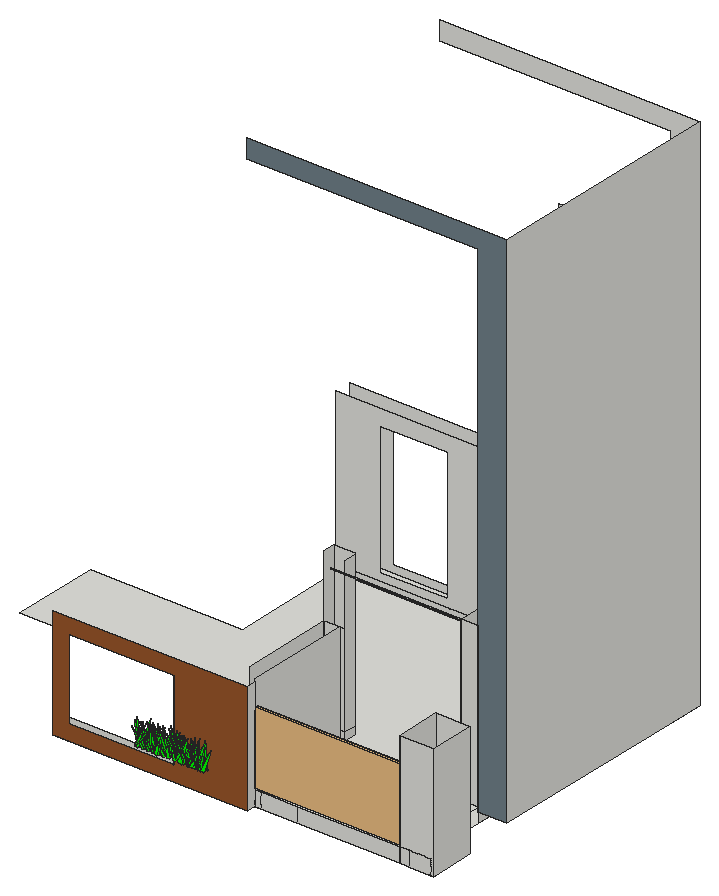
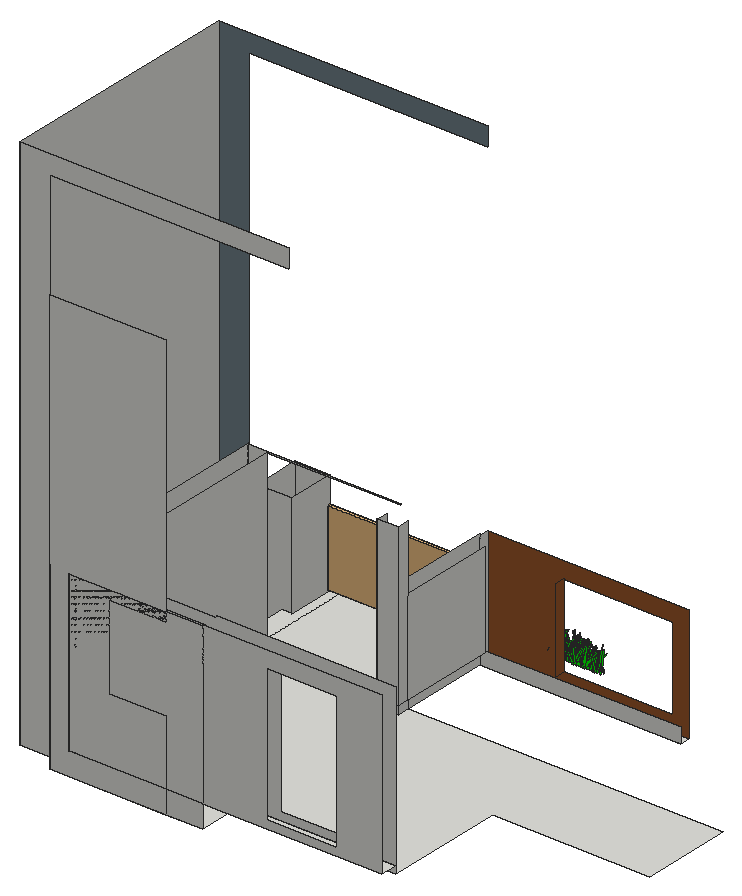
# SketchUp Ruby script. Lengths in inches.
U = 1.inch
M = Sketchup.active_model
def pt(a) = Geom::Point3d.new(a.map { |v| v * U })
def face(e, loops, mat)
  f = e.add_face(loops[0].map { |a| pt(a) })
  loops[1..].each { |l| e.add_face(l.map { |a| pt(a) }).erase! }
  f.material = f.back_material = mat if mat
  f
end
# faces: each face lists its corners as indices into pts; further lists are holes
def faces(e, pts, list, mat = nil) = list.each { |f| face(e, (f[0].is_a?(Array) ? f : [f]).map { |l| l.map { |i| pts[i] } }, mat) }
# xy, xz, yz: faces in a plane at the given z, y or x. An outline is a flat list of corners, or four numbers for a rectangle; further outlines are holes
def ring(l) = l.size == 4 ? [[l[0], l[1]], [l[2], l[1]], [l[2], l[3]], [l[0], l[3]]] : l.each_slice(2).to_a
def flat(e, list, mat, &to3) = list.each { |f| face(e, (f[0].is_a?(Array) ? f : [f]).map { |l| ring(l).map { |u, v| to3.(u, v) } }, mat) }
def xy(e, z, list, mat = nil) = flat(e, list, mat) { |x, y| [x, y, z] }
def xz(e, y, list, mat = nil) = flat(e, list, mat) { |x, z| [x, y, z] }
def yz(e, x, list, mat = nil) = flat(e, list, mat) { |y, z| [x, y, z] }
def lines(e, pts, list) = list.each { |a, b| e.add_line(pt(pts[a]), pt(pts[b])) }
# prism: a flat outline (further loops are holes) pulled along v
def prism(e, loops, v, mat = nil)
  f = face(e, loops, mat); d = Geom::Vector3d.new(v.map { |x| x * U })
  f.pushpull(f.normal.samedirection?(d) ? d.length : -d.length)
end
def box(e, o, s, mat = nil) = prism(e, [[o, [o[0] + s[0], o[1], o[2]], [o[0] + s[0], o[1] + s[1], o[2]], [o[0], o[1] + s[1], o[2]]]], [0, 0, s[2]], mat)
def at(x, y, z, deg = 0) = Geom::Transformation.translation(pt([x, y, z])) * Geom::Transformation.rotation(ORIGIN, Z_AXIS, deg.degrees)
def axes(o, x, y, z) = Geom::Transformation.new([*x, 0, *y, 0, *z, 0, *pt(o).to_a, 1])
def part(name) = M.definitions.add(name)
# library, detail: a bought-in or finely detailed component or shape, given as its bounding box
def library(name, o, s) = part(name).tap { |d| box(d.entities, o, s) }
def detail(e, o, s) = box(e.add_group.entities, o, s)
def put(e, d, t, mat = nil) = e.add_instance(d, t).tap { |i| i.material = mat if mat }
def group(e, t, mat = nil) = e.add_group.tap { |g| g.transformation = t; g.material = mat if mat }.entities
root = M.entities
M.materials.add("[0065_Lime]").color = [0, 255, 0]
M.materials.add("[0111_SlateGray]1").color = [112, 128, 136]
M.materials.add("[Wood Cherry Original]").color = [152, 86, 42]
c1 = part("fur_instance\#9")
p = [[0.8125,0,1.79],[0.67,-0.02,1.48],[0,-0.11,0],[0,0.11,0]]
faces(c1.entities,p,[[0,1,2,3]])
c2 = library("Modern+Gate+1",[0,0,0],[118.11,1.97,78.74])
xy(root,-11.8125,[[187.77,39.75,190.59,97.05],[190.59,39.75,210.17,217.05],[210.17,39.75,210.17,217.05,270.7,217.05,270.7,64.5,265.92,64.5,265.92,39.75],[265.92,39.75,270.7,64.5],[270.7,39.75,284.23,64.5]])
xy(root,-11.6,[[82.49,34.4375,187.77,39.75]])
xy(root,-6,[[270.7,86.99,286.33,217.05]])
xy(root,-3.9375,[[187.77,39.75,260.82,39.75,260.82,208.05,96.96,208.05,96.96,144.8,14.71,144.8,14.71,97.05,179.21,97.05,179.21,103.41,190.59,103.41,190.59,97.05,187.77,97.05],[260.82,39.75,270.7,87.55]])
xy(root,0,[[179.21,97.05,190.59,103.41],[96.96,208.05,190.59,217.05],[190.59,208.05,260.82,217.05]])
xz(root,34.4375,[[[82.49,-11.6,187.77,48.65],[90.86,-3.22,147.74,40.28]]],"[Wood Cherry Original]")
xz(root,39.75,[[187.77,-11.8125,190.59,-3.9375],[190.59,-11.8125,210.17,-3.9375],[210.17,-11.8125,265.92,-3.9375],[265.92,-11.8125,270.7,-3.9375],[282.96,-11.8125,284.23,-11.8125,284.23,49.9375,265.92,49.9375,265.92,-3.9375,282.96,-3.9375],
  [270.7,-11.8125,282.96,-3.9375],[82.49,-11.6,187.77,-3.9375]])
xz(root,64.5,[[265.92,-11.8125,284.23,49.9375]])
xz(root,86.99,[[270.7,-6,286.33,-6,286.33,276.75,145.58,276.75,145.58,266.9,270.7,266.9]],"[0111_SlateGray]1")
xz(root,87.55,[[260.82,-3.9375,270.7,-3.9375,270.7,84,190.59,84,190.59,83.3,260.82,83.3]])
xz(root,97.05,[[187.77,-11.8125,190.59,-3.9375],[187.77,-3.9375,190.59,0],[179.21,0,187.77,49.9375],[187.77,0,190.59,49.9375]])
xz(root,103.41,[[179.21,-3.9375,190.59,0],[179.21,0,190.59,84]])
xz(root,208.05,[[96.96,-3.9375,190.59,0],[190.59,-3.9375,260.82,0],[[96.96,0,260.82,0,260.82,83.3,190.59,83.3,190.59,84,96.96,84],[120.48,4.04,157.11,75.48],[195.64,34.28,239.77,78.41]]])
xz(root,217.05,[[190.59,-11.8125,210.17,0],[210.17,-11.8125,210.17,0,260.82,0,260.82,83.3,210.17,83.3,210.17,210.6875,270.7,210.6875,270.7,-11.8125],[270.7,-6,270.7,266.9,145.58,266.9,145.58,276.75,286.33,276.75,286.33,-6],[[96.96,0,190.59,84],[120.48,4.04,157.11,75.48]],[190.59,0,260.82,83.3],
  [210.17,0,210.17,34.28,239.77,34.28,239.77,78.41,210.17,78.41,210.17,83.3,260.82,83.3,260.82,0]])
yz(root,147.74,[[34.4375,-3.22,39.75,40.28]],"[Wood Cherry Original]")
yz(root,179.21,[[97.05,-3.9375,103.41,0],[46.62,0,97.05,49.9375],[97.05,0,103.41,84]])
yz(root,187.77,[[39.75,-11.8125,97.05,-3.9375],[34.4375,-11.6,39.75,48.65],[39.75,-3.9375,97.05,49.9375]])
yz(root,190.59,[[97.05,-3.9375,103.41,0],[97.05,0,103.41,83.3]])
yz(root,260.82,[[87.55,-3.9375,208.05,83.3],[208.05,0,217.05,83.3]])
yz(root,265.92,[[39.75,-11.8125,64.5,49.9375]])
yz(root,270.7,[[87.55,-11.8125,217.05,-6],[86.99,-6,217.05,-6,217.05,84,87.55,84,87.55,-3.9375,86.99,-3.9375],[86.99,-3.9375,87.55,84]])
yz(root,284.23,[[39.75,-11.8125,64.5,49.9375]])
yz(root,286.33,[[86.99,-6,217.05,276.75]])
put(root,c1,axes([131.16,30.08,1.48],[1.34479,0.85676,0.05361],[-5.98551,0.18367,0.98068],[1.16348,-0.04536,4.98315]),"[0065_Lime]")
put(root,c1,axes([154.34,30.49,1.48],[3.14543,1.05905,2.9173],[-8.27321,0.32433,1.95662],[1.10444,-0.58664,6.34829]),"[0065_Lime]")
put(root,c1,axes([151.13,30.3,1.48],[1.80183,0.66729,0.2231],[-4.17247,0.20193,2.05746],[2.28398,-0.15752,3.58266]),"[0065_Lime]")
put(root,c1,axes([145.91,30.29,1.48],[-2.59905,0.85083,0.56619],[-5.79357,-0.31187,-1.89204],[-1.89246,-0.21373,5.01467]),"[0065_Lime]")
put(root,c1,axes([159.01,30.73,1.48],[-6.63318,-0.16004,0.14386],[1.05389,-0.90093,-1.4343],[0.46672,-0.24023,5.28324]),"[0065_Lime]")
put(root,c1,axes([142.71,30.08,1.48],[7.1215,0.64622,0.85917],[-4.2586,0.99595,-1.74641],[-2.03213,0.17751,6.67076]),"[0065_Lime]")
put(root,c1,axes([141.75,29.98,1.48],[-3.22411,1.01338,0.01102],[-6.84097,-0.43041,2.02923],[2.28272,0.14142,6.09685]),"[0065_Lime]")
put(root,c1,axes([164.13,30.39,1.48],[-9.11333,-0.22585,0.06186],[1.59055,-1.25512,1.48409],[-0.24348,0.25431,7.37956]),"[0065_Lime]")
put(root,c1,axes([158.55,30.76,1.48],[-5.14463,0.33477,0.55676],[-2.38746,-0.60963,-2.31346],[-0.66652,-0.40025,3.98935]),"[0065_Lime]")
put(root,c1,axes([156.43,30.75,1.48],[-6.69144,-0.10778,0.79677],[0.55783,-0.93298,-1.12936],[1.11205,-0.18053,5.36088]),"[0065_Lime]")
put(root,c1,axes([155.84,30.42,1.48],[2.12265,0.71652,0.65154],[-5.08256,0.26891,1.04616],[0.90042,-0.17123,4.36925]),"[0065_Lime]")
put(root,c1,axes([131.06,30.3,1.48],[6.03432,-0.06931,0.12824],[0.51555,0.78005,-1.92468],[0.04819,0.33316,4.53309]),"[0065_Lime]")
put(root,c1,axes([139.76,30.26,1.48],[4.28673,0.42625,0.07193],[-2.89396,0.58065,-1.18856],[-0.91349,0.16073,4.10291]),"[0065_Lime]")
put(root,c1,axes([134.27,30.65,1.48],[-5.47557,0.46539,0.18725],[-3.19592,-0.72199,-1.70432],[-0.899,-0.2679,4.91834]),"[0065_Lime]")
put(root,c1,axes([164.87,30.92,1.48],[-5.23437,-0.7374,2.64853],[4.53926,-0.86605,-2.14421],[4.18761,0.01704,5.63483]),"[0065_Lime]")
put(root,c1,axes([147.65,31.12,1.48],[-0.61701,-1.22551,0.08673],[8.43304,-0.07999,1.82147],[-2.22661,0.03665,6.87461]),"[0065_Lime]")
put(root,c1,axes([137.36,30.65,1.48],[-2.94014,0.52007,0.68147],[-3.72191,-0.36617,-1.26052],[-0.74,-0.22464,3.63235]),"[0065_Lime]")
put(root,c1,axes([136.8,30.66,1.48],[-2.24611,0.64016,1.05541],[-4.57918,-0.2418,-1.53336],[-1.21228,-0.27275,3.83655]),"[0065_Lime]")
put(root,c1,axes([163.99,30.5,1.48],[7.7081,-0.00024,2.91079],[0.63982,1.175,-1.11785],[-3.52083,0.21301,6.16942]),"[0065_Lime]")
put(root,c1,axes([139.59,30.46,1.48],[7.86284,0.00707,1.28311],[0.31298,1.09698,-1.47145],[-1.54689,0.25787,6.2243]),"[0065_Lime]")
put(root,c1,axes([144.19,30.66,1.48],[1.09152,0.53515,0.77575],[-3.71155,0.09531,1.25204],[1.27983,-0.18,2.96936]),"[0065_Lime]")
put(root,c1,axes([144.24,30.89,1.48],[-4.88102,0.10111,0.10384],[-0.72599,-0.6571,-1.13982],[-0.08333,-0.19737,3.84792]),"[0065_Lime]")
put(root,c1,axes([140.92,30.625,1.48],[-0.10932,1.03791,1.64047],[-7.42428,0.05493,-1.49191],[-1.87214,-0.27844,5.82061]),"[0065_Lime]")
put(root,c1,axes([160.6,31.19,1.48],[-3.82499,-0.52984,0.36441],[3.26372,-0.50442,-1.90954],[1.94073,-0.19599,3.92948]),"[0065_Lime]")
put(root,c1,axes([147.97,30.61,1.48],[2.56392,1.18106,2.50526],[-8.42978,0.47002,-1.71695],[-3.0117,-0.31013,6.93855]),"[0065_Lime]")
put(root,c1,axes([143.21,31.14,1.48],[-0.13594,-0.86218,0.22063],[5.90466,-0.00786,1.37836],[-1.69,0.0419,4.79808]),"[0065_Lime]")
put(root,c1,axes([164.19,31.2,1.48],[8.11735,-0.23094,2.64105],[0.74681,1.19725,1.98942],[-3.56168,-0.2753,6.43629]),"[0065_Lime]")
put(root,c1,axes([151.46,31.14,1.48],[7.34316,-0.34163,1.5518],[2.12221,1.05982,1.17389],[-2.24647,-0.1155,6.18141]),"[0065_Lime]")
put(root,c1,axes([166.45,30.57,1.48],[1.17382,1.09024,0.44262],[-7.59312,0.14388,1.44791],[1.68497,-0.11114,6.21651]),"[0065_Lime]")
put(root,c1,axes([155.1875,30.54,1.48],[7.07469,0.25889,0.42712],[-1.57252,0.946,-1.98005],[-1.09419,0.31433,5.60725]),"[0065_Lime]")
put(root,c1,axes([130.35,31.05,1.48],[6.37414,0.19571,0.84766],[-1.59783,0.8786,1.15247],[-0.68751,-0.22748,5.18049]),"[0065_Lime]")
put(root,c1,axes([136.87,30.85,1.48],[-4.20883,-0.27554,0.19585],[1.92038,-0.55188,1.28727],[-0.46406,0.21528,3.55071]),"[0065_Lime]")
put(root,c1,axes([151.14,30.7,1.48],[-6.44363,0.24769,0.74746],[-1.48744,-0.89136,1.4137],[1.31873,0.20488,5.24679]),"[0065_Lime]")
put(root,c1,axes([138.02,31.46,1.48],[-5.96483,-0.81292,0.95816],[5.29838,-0.84088,-2.08212],[2.6044,-0.15114,6.43034]),"[0065_Lime]")
put(root,c1,axes([164.6,30.84,1.48],[-3.07447,0.90372,1.06173],[-6.54392,-0.40698,-0.92984],[-0.49282,-0.23377,5.72331]),"[0065_Lime]")
put(root,c1,axes([160.23,30.6,1.48],[8.1239,-0.2781,1.33211],[2.53508,0.99126,-3.29473],[-0.41505,0.61115,5.95006]),"[0065_Lime]")
put(root,c1,axes([142.43,30.93,1.48],[-7.15382,-0.24663,1.73765],[2.14008,-1.02115,0.97289],[1.75045,0.24053,5.91207]),"[0065_Lime]")
put(root,c1,axes([148.04,31.38,1.48],[6.36239,-0.63633,1.08188],[4.24364,0.90857,1.39483],[-2.06583,-0.09341,6.19726]),"[0065_Lime]")
put(root,c1,axes([162.57,30.92,1.48],[5.10738,0.02077,0.30646],[-0.05531,0.69972,-0.9794],[-0.40092,0.16809,4.0391]),"[0065_Lime]")
put(root,c1,axes([155.83,31.41,1.48],[6.62755,-0.4728,1.829],[2.75521,0.97124,1.80736],[-2.96415,-0.15437,5.76943]),"[0065_Lime]")
put(root,c1,axes([158.45,30.86,1.48],[-3.32497,1.04784,0.37862],[-7.25967,-0.43616,-1.73353],[-1.76663,-0.17982,6.41105]),"[0065_Lime]")
put(root,c1,axes([156.64,31.38,1.48],[0.69433,-1.01539,1.19312],[7.09847,0.14806,1.48899],[-1.99475,0.17344,5.71402]),"[0065_Lime]")
put(root,c1,axes([158.63,31.03,1.48],[6.87786,-0.04923,0.77182],[0.52152,0.95779,-1.02778],[-0.86667,0.18566,5.5067]),"[0065_Lime]")
put(root,c1,axes([141.43,31.07,1.48],[5.92325,-0.20071,0.50734],[1.55104,0.793,-1.46875],[-0.15359,0.26757,4.73353]),"[0065_Lime]")
put(root,c1,axes([137.89,31.49,1.48],[5.56421,-0.34651,0.72564],[2.25126,0.78199,1.09112],[-1.34485,-0.12463,4.82882]),"[0065_Lime]")
put(root,c1,axes([165.58,31.19,1.48],[-1.509,0.69969,1.01747],[-4.74864,-0.12057,-1.8814],[-1.95166,-0.24763,3.79099]),"[0065_Lime]")
put(root,c1,axes([159.92,31.53,1.48],[-3.81317,-0.7006,0.80758],[4.85423,-0.55358,-0.92775],[1.51033,0.0104,5.0207]),"[0065_Lime]")
put(root,c1,axes([139.42,30.93,1.48],[6.64759,0.5258,2.30818],[-3.01847,1.0078,-1.941],[-3.59757,0.12599,5.89361]),"[0065_Lime]")
put(root,c1,axes([161.58,30.86,1.48],[-5.36162,0.57347,0.33359],[-3.82513,-0.73332,1.5654],[1.4805,0.18213,5.25257]),"[0065_Lime]")
put(root,c1,axes([159.25,31.44,1.48],[3.91816,-0.87225,2.52622],[6.06539,0.67392,1.5729],[-3.3747,0.19852,5.76003]),"[0065_Lime]")
put(root,c1,axes([145.25,31.25,1.48],[-6.42762,-0.82405,2.16233],[6.35104,-0.89824,1.02041],[1.05919,0.3853,7.00345]),"[0065_Lime]")
put(root,c1,axes([151.1,31.56,1.48],[-8.31821,0.11653,0.23198],[-0.87696,-1.10569,-2.19415],[0.00085,-0.38115,6.43594]),"[0065_Lime]")
put(root,c1,axes([131.46,31.08,1.48],[5.54293,-0.08125,2.31221],[1.41685,0.82754,-1.27283],[-2.53126,0.28528,4.3508]),"[0065_Lime]")
put(root,c1,axes([137.3,31.63,1.48],[1.75748,-0.68829,0.18629],[4.58809,0.24288,1.43112],[-1.73043,-0.05507,3.98371]),"[0065_Lime]")
put(root,c1,axes([135.01,31.5625,1.48],[-6.15,0.03221,1.76329],[-0.79479,-0.88215,-1.29408],[2.0298,-0.24781,4.8358]),"[0065_Lime]")
put(root,c1,axes([154.8,31.43,1.48],[-6.90066,-0.87302,0.88249],[6.26072,-0.92092,1.86334],[-0.76182,0.3397,7.31943]),"[0065_Lime]")
put(root,c1,axes([161.17,31.36,1.48],[-4.13046,1.11656,1.37914],[-7.71419,-0.45502,-2.9419],[-2.55069,-0.43195,6.66403]),"[0065_Lime]")
put(root,c1,axes([134.28,30.85,1.48],[4.4557,1.01846,0.24991],[-6.6833,0.596,-2.54936],[-2.8213,0.1966,6.4338]),"[0065_Lime]")
put(root,c1,axes([162.76,31.37,1.48],[4.62723,1.01985,1.80873],[-7.58747,0.61052,1.30775],[0.2258,-0.38427,6.87815]),"[0065_Lime]")
put(root,c1,axes([135.6,31.78,1.48],[8.1008,-0.1572,1.83452],[0.48244,1.145,1.87817],[-2.47089,-0.29181,6.38117]),"[0065_Lime]")
put(root,c1,axes([133.4,31.43,1.48],[-1.66271,-0.52795,1.16072],[3.87968,-0.15421,1.32683],[-1.04904,0.26649,3.06733]),"[0065_Lime]")
put(root,c1,axes([131.49,31.02,1.48],[2.30582,1.08255,0.41825],[-7.27396,0.32986,-2.07577],[-2.58958,0.03739,6.20312]),"[0065_Lime]")
put(root,c1,axes([140.92,31.84,1.48],[9.15713,0.02109,1.33156],[-0.62912,1.24769,2.20042],[-1.51872,-0.3897,7.11713]),"[0065_Lime]")
put(root,c1,axes([144.37,31.02,1.48],[7.57589,0.60189,0.04648],[-4.11575,1.02722,-1.88416],[-1.18803,0.27953,6.82376]),"[0065_Lime]")
put(root,c1,axes([144.97,31.68,1.48],[0.52815,-0.6201,0.73916],[4.38631,0.04138,-0.91045],[1.02985,0.14178,3.49869]),"[0065_Lime]")
put(root,c1,axes([154.08,31.53,1.48],[-2.14862,0.79256,1.23868],[-5.44922,-0.18966,-2.18753],[-2.10659,-0.31776,4.39521]),"[0065_Lime]")
put(root,c1,axes([135.89,31.67,1.48],[4.78353,-1.05133,1.0815],[7.40471,0.59527,-2.27924],[1.70749,0.36382,6.85433]),"[0065_Lime]")
put(root,c1,axes([137.34,31.84,1.48],[-0.05126,-1.22547,1.67463],[8.56481,-0.09175,-2.07637],[2.63435,0.27445,6.78329]),"[0065_Lime]")
put(root,c1,axes([163.15,31.75,1.48],[2.10149,-0.48926,0.98971],[3.30454,0.33716,0.94258],[-1.63821,0.05248,3.17093]),"[0065_Lime]")
put(root,c1,axes([164.14,31.88,1.48],[-4.77978,0.01871,1.47415],[-0.67524,-0.68359,-1.15791],[1.68707,-0.2206,3.71309]),"[0065_Lime]")
put(root,c1,axes([156.09,32.22,1.48],[4.49113,-0.59291,0.32605],[3.4317,0.55683,2.65515],[-2.48758,-0.30228,4.25153]),"[0065_Lime]")
put(root,c1,axes([145.8,31.59,1.48],[-6.78697,-0.22687,0.61193],[1.76366,-0.9142,1.58517],[0.24914,0.29144,5.44877]),"[0065_Lime]")
put(root,c1,axes([157.21,32.07,1.48],[7.06815,-0.04142,1.18644],[-0.06821,0.9848,1.42091],[-1.48652,-0.24213,5.57614]),"[0065_Lime]")
put(root,c1,axes([151.2,32.07,1.48],[6.80428,-0.01169,1.86976],[-0.30445,0.99516,0.94159],[-2.27992,-0.16778,5.45443]),"[0065_Lime]")
put(root,c1,axes([156.54,32,1.48],[-5.28763,0.25256,0.49209],[-1.89335,-0.71744,-1.12209],[0.10848,-0.21111,4.40196]),"[0065_Lime]")
put(root,c1,axes([153.14,31.95,1.48],[4.1326,-0.64356,0.17073],[4.23032,0.51994,-2.07559],[1.76755,0.26028,4.56838]),"[0065_Lime]")
put(root,c1,axes([164.85,31.71,1.48],[0.00098,0.71377,0.28891],[-4.85918,0.01505,-1.23491],[-1.52196,-0.04759,3.94291]),"[0065_Lime]")
put(root,c1,axes([167.01,32.13,1.48],[4.31989,-0.07009,0.94174],[0.19122,0.61045,0.94209],[-1.24606,-0.14932,3.40943]),"[0065_Lime]")
put(root,c1,axes([143.67,32.19,1.48],[6.97103,-0.44992,2.16503],[2.98781,1.04853,0.93625],[-2.89986,-0.00123,6.1692]),"[0065_Lime]")
put(root,c1,axes([157.22,32.27,1.48],[3.96253,-0.32653,0.24837],[2.19065,0.54596,0.92739],[-0.83317,-0.11748,3.61961]),"[0065_Lime]")
put(root,c1,axes([147.21,31.89,1.48],[4.6761,-0.2114,0.94885],[1.8249,0.62155,-1.31006],[-0.54207,0.26886,3.77474]),"[0065_Lime]")
put(root,c1,axes([128.97,31.8,1.48],[8.27121,0.14008,0.09896],[-0.95467,1.14074,-1.31316],[-0.31168,0.22324,6.64815]),"[0065_Lime]")
put(root,c1,axes([139.73,32.43,1.48],[-2.51936,-0.91159,0.56912],[6.22301,-0.36737,-1.49139],[1.96209,-0.00533,5.46088]),"[0065_Lime]")
put(root,c1,axes([152.12,32.44,1.48],[-6.41238,-0.11396,1.50385],[-0.02568,-0.86041,-2.2573],[2.01871,-0.37294,4.74822]),"[0065_Lime]")
put(root,c1,axes([163.86,32.27,1.48],[-1.08146,-1.07601,1.29202],[7.58387,-0.08929,1.70829],[-1.90915,0.25483,6.0541]),"[0065_Lime]")
put(root,c1,axes([159.34,32.16,1.48],[-3.97371,-0.86449,0.60456],[5.86218,-0.48418,2.2941],[-2.00913,0.29709,5.49794]),"[0065_Lime]")
put(root,c1,axes([141.43,32.04,1.48],[-5.42476,-0.89754,1.65261],[6.64051,-0.66976,2.23354],[-0.91097,0.4626,6.44019]),"[0065_Lime]")
put(root,c1,axes([131.51,32.37,1.48],[1.6072,-1.13707,1.56242],[8.13297,0.27237,1.10671],[-1.73927,0.22287,6.61884]),"[0065_Lime]")
put(root,c1,axes([148.99,32.27,1.48],[6.40985,0.036,1.20623],[-0.52493,0.90791,0.93767],[-1.41036,-0.17431,5.13308]),"[0065_Lime]")
put(root,c1,axes([156.16,32.54,1.48],[4.49811,-0.71129,0.39345],[4.87298,0.62889,1.23723],[-1.45297,-0.09282,5.36745]),"[0065_Lime]")
put(root,c1,axes([148.26,32.43,1.48],[3.36747,-0.33135,0.40386],[2.04071,0.45588,1.27496],[-1.28159,-0.14473,3.09134]),"[0065_Lime]")
put(root,c1,axes([146.83,32.16,1.48],[-7.14365,-0.6499,0.90369],[4.75512,-0.96876,1.52509],[-0.11794,0.30579,6.75217]),"[0065_Lime]")
put(root,c1,axes([148.22,31.92,1.48],[8.77061,0.12087,0.96092],[-0.54961,1.20871,-1.77564],[-1.35404,0.29231,6.94496]),"[0065_Lime]")
put(root,c1,axes([137.6,32.55,1.48],[7.55156,0.39776,1.55121],[-3.38059,0.96126,2.6295],[-0.47003,-0.52325,6.00982]),"[0065_Lime]")
put(root,c1,axes([154.8125,32.17,1.48],[-3.7647,0.6752,0.27026],[-4.68765,-0.5,-1.34567],[-1.10694,-0.17896,4.77945]),"[0065_Lime]")
put(root,c1,axes([138.48,32.65,1.48],[5.27219,-0.06661,0.32297],[0.29641,0.69259,1.58498],[-0.54267,-0.26883,4.00343]),"[0065_Lime]")
put(root,c1,axes([136.47,32.79,1.48],[-3.43441,-0.90156,1.1985],[5.77943,-0.52474,-2.26943],[3.1519,-0.02018,5.46722]),"[0065_Lime]")
put(root,c1,axes([155.02,32.47,1.48],[-2.33121,-1.13882,2.3339],[8.30625,-0.19054,2.37393],[-2.2185,0.48328,6.43573]),"[0065_Lime]")
put(root,c1,axes([141.13,32.31,1.48],[-0.4966,0.68944,1.12791],[-4.75715,-0.13309,1.34027],[1.83452,-0.1585,3.78082]),"[0065_Lime]")
put(root,c1,axes([147.32,32.01,1.48],[7.44968,0.40387,0.06367],[-2.71252,0.99734,-1.9975],[-0.95346,0.31819,6.18023]),"[0065_Lime]")
put(root,c1,axes([140.04,32.31,1.48],[-4.84614,-0.63045,2.52701],[5.34328,-0.66683,1.20518],[1.1092,0.45785,5.23495]),"[0065_Lime]")
put(root,c1,axes([143.89,32.1,1.48],[4.16284,0.50161,0.40389],[-3.00781,0.54224,-2.05474],[-1.98566,0.23024,3.95919]),"[0065_Lime]")
put(root,c1,axes([157.07,32.81,1.48],[-4.47405,-0.26538,0.11664],[1.76364,-0.60257,-1.18013],[0.69054,-0.18042,3.76979]),"[0065_Lime]")
put(root,c1,axes([160.94,32.29,1.48],[0.23644,1.10069,1.29161],[-7.82687,0.07709,-1.25327],[-1.61833,-0.21201,6.25003]),"[0065_Lime]")
put(root,c1,axes([152.16,32.84,1.48],[3.33577,-0.72041,1.14417],[4.76403,0.50863,1.54157],[-2.35938,0.00849,4.73038]),"[0065_Lime]")
put(root,c1,axes([147.56,32.74,1.48],[-3.64666,-0.71529,0.22588],[4.96102,-0.48686,1.32943],[-1.17383,0.1645,4.9169]),"[0065_Lime]")
put(root,c1,axes([152.72,32.16,1.48],[2.26642,1.2277,0.63083],[-8.49416,0.33527,-1.67281],[-2.18758,-0.02988,7.14889]),"[0065_Lime]")
put(root,c1,axes([152.7,32.22,1.48],[-5.02569,0.9045,0.21849],[-6.25566,-0.69657,1.42218],[1.54033,0.12221,6.48869]),"[0065_Lime]")
put(root,c1,axes([167.45,33.05,1.48],[-7.46944,0.2291,0.12301],[-1.52502,-0.93724,-2.77757],[-0.59615,-0.47294,5.56404]),"[0065_Lime]")
put(root,c1,axes([150.04,32.96,1.48],[-4.2878,-0.21134,0.6611],[1.17728,-0.58863,-1.25338],[1.23962,-0.172,3.47709]),"[0065_Lime]")
put(root,c1,axes([154.41,32.99,1.48],[6.33569,-0.15796,0.85918],[0.84566,0.88044,1.29799],[-1.29004,-0.19862,5.07052]),"[0065_Lime]")
put(root,c1,axes([160.43,32.55,1.48],[6.05181,-0.32335,1.11798],[2.65612,0.78747,-1.8811],[-0.3597,0.37463,4.91906]),"[0065_Lime]")
put(root,c1,axes([166.02,33.14,1.48],[-8.26026,-0.01836,3.45578],[-1.26025,-1.2355,-2.21302],[4.05937,-0.42092,6.34499]),"[0065_Lime]")
put(root,c1,axes([150.11,32.72,1.48],[-4.09216,-0.71838,1.43924],[5.34677,-0.48958,1.87008],[-0.82392,0.39087,4.98751]),"[0065_Lime]")
put(root,c1,axes([132.875,33.23,1.48],[4.89678,-0.68978,0.44492],[4.52046,0.66948,1.8621],[-1.9904,-0.17652,5.32366]),"[0065_Lime]")
put(root,c1,axes([131.22,33.07,1.48],[5.13047,-0.22405,0.97399],[1.21707,0.71977,1.30631],[-1.57949,-0.17313,4.17027]),"[0065_Lime]")
put(root,c1,axes([140.8,33.42,1.48],[3.28074,-1.09396,0.49555],[7.10675,0.45675,2.65725],[-3.2364,-0.10597,6.33734]),"[0065_Lime]")
put(root,c1,axes([138.46,33.34,1.48],[2.37141,-0.99867,0.13924],[6.89721,0.32934,1.43178],[-1.72282,-0.05613,5.92372]),"[0065_Lime]")
put(root,c1,axes([164.66,33.1875,1.48],[-4.72687,0.03757,0.04958],[-0.25893,-0.56287,-2.04265],[-0.09021,-0.35274,3.26468]),"[0065_Lime]")
put(root,c1,axes([163.52,33.04,1.48],[4.68373,-0.737,0.08541],[5.09533,0.63442,-1.43469],[1.24802,0.17575,5.5369]),"[0065_Lime]")
put(root,c1,axes([163.38,32.8,1.48],[1.92301,0.52632,1.14527],[-3.59359,0.3237,-0.99248],[-1.76001,-0.08588,3.27779]),"[0065_Lime]")
put(root,c1,axes([143.18,33.15,1.48],[-1.70349,-0.54913,0.77525],[3.62071,-0.27269,-1.20835],[1.75237,0.0296,3.2503]),"[0065_Lime]")
put(root,c1,axes([138.52,32.8,1.48],[-4.11719,0.92635,0.10528],[-6.09933,-0.52692,-2.46248],[-2.50492,-0.23958,5.82293]),"[0065_Lime]")
put(root,c1,axes([161.04,33.26,1.48],[-3.64972,-1.08612,0.37877],[7.50988,-0.47885,1.86725],[-1.88736,0.19493,6.69743]),"[0065_Lime]")
put(root,c1,axes([150.97,33.09,1.48],[-3.37064,-1.16113,2.21965],[8.69398,-0.43151,1.17123],[-0.37703,0.4303,7.16399]),"[0065_Lime]")
put(root,c1,axes([134.21,33.19,1.48],[0.25834,-0.98164,1.45104],[7.09045,0.08009,0.98038],[-1.30798,0.24029,5.60117]),"[0065_Lime]")
put(root,c1,axes([138.85,33.26,1.48],[-4.17903,-0.24254,1.60705],[1.09667,-0.63585,-1.32873],[2.38325,-0.1327,3.4294]),"[0065_Lime]")
put(root,c1,axes([142.08,32.85,1.48],[-2.33256,0.77265,0.09252],[-5.29724,-0.31096,-1.34396],[-1.47864,-0.10482,4.66881]),"[0065_Lime]")
put(root,c1,axes([166.02,32.9,1.48],[2.21853,0.50046,0.68876],[-3.19532,0.33262,-1.2887],[-1.78642,0.02656,3.16042]),"[0065_Lime]")
put(root,c1,axes([139.85,33.05,1.48],[-4.30085,-0.10806,1.33851],[1.29437,-0.59929,1.13054],[1.2743,0.24402,3.36924]),"[0065_Lime]")
put(root,c1,axes([133.83,32.97,1.48],[-5.91086,0.44805,0.45225],[-3.06965,-0.82759,0.92921],[1.02642,0.10521,5.38332]),"[0065_Lime]")
put(root,c1,axes([145.92,33.22,1.48],[6.27301,0.75513,0.59973],[-5.40287,0.8558,1.28346],[0.481,-0.23521,6.59516]),"[0065_Lime]")
put(root,c1,axes([157.4,33.42,1.48],[8.34097,0.36053,1.12891],[-2.8001,1.15516,1.3265],[-0.81767,-0.27811,6.97334]),"[0065_Lime]")
put(root,c1,axes([142.31,33.25,1.48],[-7.90002,-0.29151,1.02764],[2.2589,-1.10378,0.99775],[0.89283,0.21327,6.5685]),"[0065_Lime]")
put(root,c1,axes([150.43,33.33,1.48],[3.51533,-0.54853,0.79412],[3.96203,0.44002,-1.41957],[0.70287,0.26307,4.03033]),"[0065_Lime]")
put(root,c1,axes([143.8125,33.35,1.48],[-5.49328,-0.69024,0.93571],[5.00166,-0.71385,1.78273],[-0.65989,0.33522,5.72295]),"[0065_Lime]")
put(root,c1,axes([146.79,33.09,1.48],[-3.09962,0.61445,0.38008],[-4.17491,-0.43639,1.11308],[1.38188,0.05983,4.21535]),"[0065_Lime]")
put(root,c1,axes([155.88,33.08,1.48],[-3.07006,0.70991,0.32607],[-4.88785,-0.43216,1.07908],[1.33917,0.05012,4.68607]),"[0065_Lime]")
put(root,c1,axes([154.43,33.22,1.48],[4.21636,0.7436,1.92447],[-5.00918,0.67428,-1.46894],[-2.91709,-0.08306,5.30406]),"[0065_Lime]")
put(root,c1,axes([156.44,33.08,1.48],[6.76117,0.11583,0.24477],[-0.60698,0.85458,-2.45758],[-0.63371,0.41725,4.96545]),"[0065_Lime]")
put(root,c1,axes([159.28,32.94,1.48],[-5.33162,0.80097,0.08228],[-5.19506,-0.6906,2.54439],[2.34797,0.29077,5.8165]),"[0065_Lime]")
put(root,c1,axes([152.12,33.31,1.48],[5.56637,0.401,0.33307],[-2.70545,0.7698,-1.14016],[-0.99595,0.15006,4.95871]),"[0065_Lime]")
put(root,c1,axes([143.9,33.35,1.48],[0.35386,0.74543,0.04025],[-5.03989,0.04506,1.35276],[1.65632,-0.02214,4.10761]),"[0065_Lime]")
put(root,c1,axes([132.17,33.43,1.48],[8.33877,-0.27594,2.01499],[2.57823,1.16187,-1.72788],[-1.82907,0.37975,6.75079]),"[0065_Lime]")
put(root,c1,axes([129.41,33.45,1.48],[3.87874,0.40201,0.48741],[-2.57705,0.53634,-1.25454],[-1.37942,0.1284,3.71427]),"[0065_Lime]")
put(root,c1,axes([142.93,33.4,1.48],[4.21742,0.73133,0.67611],[-4.96635,0.60151,-1.30551],[-1.7646,0.05497,5.2902]),"[0065_Lime]")
put(root,c1,axes([160,33.47,1.48],[-4.93652,0.91988,0.64008],[-6.3138,-0.6993,1.45788],[1.89993,0.06618,6.50789]),"[0065_Lime]")
put(root,c2,axes([187.77,39.75,-3],[0.6616,0,0],[0,0.82592,0],[0,0,0.5]))
